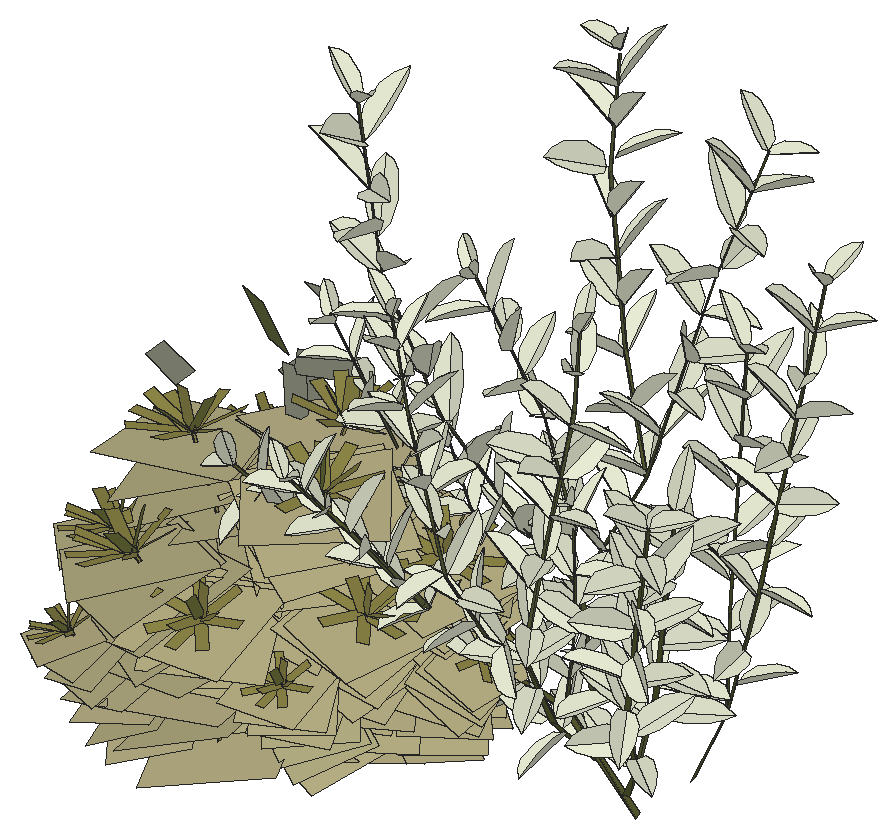
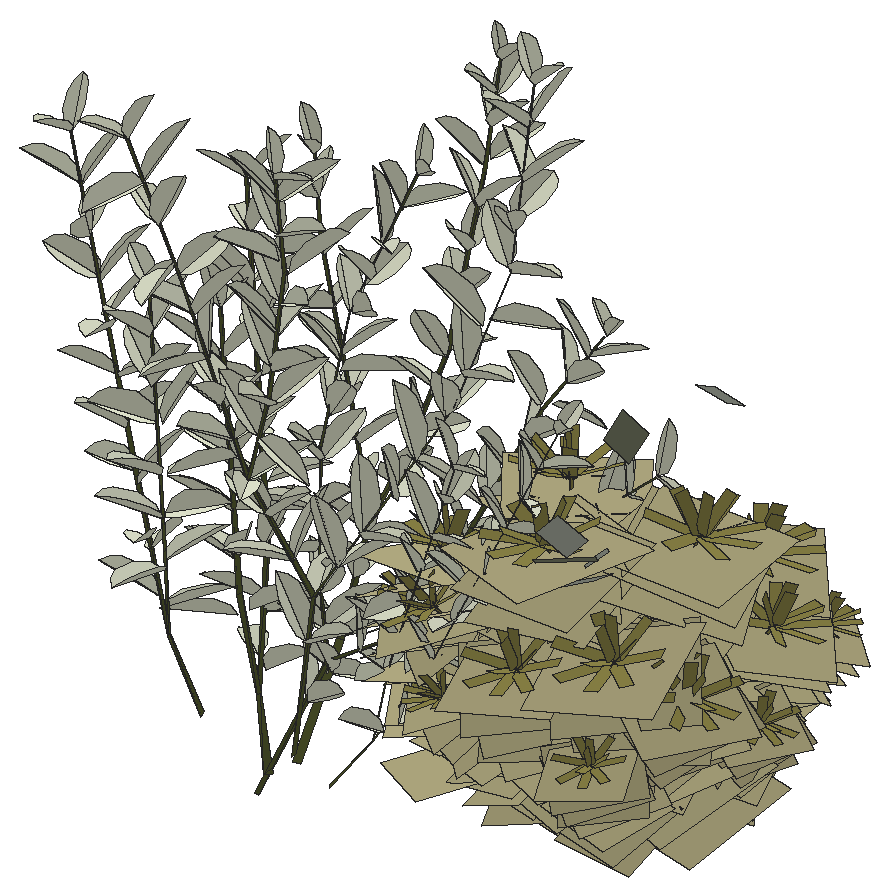
# SketchUp Ruby script. Lengths in inches.
U = 1.inch
M = Sketchup.active_model
def pt(a) = Geom::Point3d.new(a.map { |v| v * U })
def face(e, loops, mat)
  f = e.add_face(loops[0].map { |a| pt(a) })
  loops[1..].each { |l| e.add_face(l.map { |a| pt(a) }).erase! }
  f.material = f.back_material = mat if mat
  f
end
# faces: each face lists its corners as indices into pts; further lists are holes
def faces(e, pts, list, mat = nil) = list.each { |f| face(e, (f[0].is_a?(Array) ? f : [f]).map { |l| l.map { |i| pts[i] } }, mat) }
# xy, xz, yz: faces in a plane at the given z, y or x. An outline is a flat list of corners, or four numbers for a rectangle; further outlines are holes
def ring(l) = l.size == 4 ? [[l[0], l[1]], [l[2], l[1]], [l[2], l[3]], [l[0], l[3]]] : l.each_slice(2).to_a
def flat(e, list, mat, &to3) = list.each { |f| face(e, (f[0].is_a?(Array) ? f : [f]).map { |l| ring(l).map { |u, v| to3.(u, v) } }, mat) }
def xy(e, z, list, mat = nil) = flat(e, list, mat) { |x, y| [x, y, z] }
def xz(e, y, list, mat = nil) = flat(e, list, mat) { |x, z| [x, y, z] }
def yz(e, x, list, mat = nil) = flat(e, list, mat) { |y, z| [x, y, z] }
def lines(e, pts, list) = list.each { |a, b| e.add_line(pt(pts[a]), pt(pts[b])) }
# prism: a flat outline (further loops are holes) pulled along v
def prism(e, loops, v, mat = nil)
  f = face(e, loops, mat); d = Geom::Vector3d.new(v.map { |x| x * U })
  f.pushpull(f.normal.samedirection?(d) ? d.length : -d.length)
end
def box(e, o, s, mat = nil) = prism(e, [[o, [o[0] + s[0], o[1], o[2]], [o[0] + s[0], o[1] + s[1], o[2]], [o[0], o[1] + s[1], o[2]]]], [0, 0, s[2]], mat)
def at(x, y, z, deg = 0) = Geom::Transformation.translation(pt([x, y, z])) * Geom::Transformation.rotation(ORIGIN, Z_AXIS, deg.degrees)
def axes(o, x, y, z) = Geom::Transformation.new([*x, 0, *y, 0, *z, 0, *pt(o).to_a, 1])
def part(name) = M.definitions.add(name)
# library, detail: a bought-in or finely detailed component or shape, given as its bounding box
def library(name, o, s) = part(name).tap { |d| box(d.entities, o, s) }
def detail(e, o, s) = box(e.add_group.entities, o, s)
def put(e, d, t, mat = nil) = e.add_instance(d, t).tap { |i| i.material = mat if mat }
def group(e, t, mat = nil) = e.add_group.tap { |g| g.transformation = t; g.material = mat if mat }.entities
root = M.entities
M.materials.add("0ad16as01f6asdLeafVar1sfd015as60f1as6").color = [231, 235, 211]
M.materials.add("Colorsadfasdfa0sd1f06w3").color = [153, 130, 61]
M.materials.add("Euphorbia asdfasd0f150160s159w").color = [180, 173, 131]
M.materials.add("Euphorbiaasdfa0sdf1a56sd016wow Leaf SU").color = [141, 134, 72]
M.materials.add("asdfasdf0165f6asdLeafVar1sfd015as60f1as6").color = [231, 235, 211]
M.materials.add("dw_stemssadfasdfa0sdf1s01d6w1").color = [90, 97, 50]
M.materials.add("viburnumblaasdfas0df1w06d").color = [98, 102, 84]
M.materials.add("viburnumbladsadfasdfad0w122").color = [125, 129, 119]
c1 = part("Component\#315")
p = [[0.25,0,0],[2.05,0.01,0.35],[1.81,4.2,1.66],[0,4.19,1.3125]]
faces(c1.entities,p,[[0,1,2,3]],"viburnumbladsadfasdfad0w122")
c2 = part("viburnumblad2")
put(c2.entities,c1,axes([-19.23,-4.49,-32.18],[83.35428,0,0],[0,79.38502,0],[0,0,83.35428]))
c3 = part("Component\#314")
p = [[0.14,0,0],[2.58,0.05,0.25],[2.44,5.11,2.64],[0,5.05,2.39]]
faces(c3.entities,p,[[0,1,2,3]],"viburnumblaasdfas0df1w06d")
c4 = part("viburnumblad1\#2")
put(c4.entities,c3,axes([-37.25,6.23,19.31],[75.98784,0,0],[0,65.50676,0],[0,0,75.98784]))
c5 = part("Component\#306")
p = [[4.55,0.11,0],[4.55,0,0],[2.84,0,3.13],[2.84,0.11,3.13],[4.625,0.05,0.04],[2.92,0.05,3.15],
  [2.08,0,8.07],[2.08,0.11,8.07],[2.16,0.05,8.1],[0,0,12.54],[0,0.11,12.54],[0.07,0.05,12.58]]
faces(c5.entities,p,[[0,1,2,3],[1,4,5,2],[1,0,4],[4,0,3,5],[3,2,6,7],[2,5,8,6],[5,3,7,8],[7,6,9,10],
  [6,8,11,9],[8,7,10,11],[10,9,11]],"Colorsadfasdfa0sd1f06w3")
c6 = part("Component\#301")
xy(c6.entities,0,[[0,0,0.7,3.1]],"Euphorbiaasdfa0sdf1a56sd016wow Leaf SU")
c7 = part("Leaf rosette")
put(c7.entities,c6,axes([2.21,1.74,0.13],[-0.4441,0.47879,-0.0956],[-0.4878,-0.4406,0.05935],[-0.03146,0.16757,0.98536]))
put(c7.entities,c6,axes([2.29,1.9,0.17],[-0.62678,-0.10063,-0.18061],[0.01105,-0.59203,0.2915],[-0.31282,0.41486,0.85442]))
put(c7.entities,c6,axes([2.09,1.69,0.1],[-0.10438,0.65169,0],[-0.65169,-0.10438,0],[0,0,1]))
put(c7.entities,c6,axes([1.97,1.77,0.02],[0.31114,0.5228,0.25587],[-0.57125,0.32993,0.02052],[-0.16918,-0.3502,0.92127]))
put(c7.entities,c6,axes([1.93,1.95,0],[0.54816,-0.03215,0.36617],[-0.11878,0.60671,0.23108],[-0.52706,-0.39065,0.75472]))
put(c7.entities,c6,axes([2.04,2.1,0.05],[0.26275,-0.55867,0.23335],[0.34186,0.34684,0.44545],[-0.75711,-0.08556,0.64766]))
put(c7.entities,c6,axes([2.22,2.08,0.13],[-0.29265,-0.59104,-0.02512],[0.40323,-0.2198,0.47401],[-0.65583,0.2952,0.69479]))
c8 = part("Component\#308")
xy(c8.entities,0,[[0,0,5.01,4.64]],"Euphorbia asdfasd0f150160s159w")
c9 = part("Component\#316")
put(c9.entities,c5,at(2.35,3.5,0))
put(c9.entities,c7,at(0.25,1.59,12.45))
put(c9.entities,c8,axes([7.46,0.77,3.64],[0.10848,0.99337,0.03799],[-0.82378,0.11122,-0.55589],[-0.55643,0.02901,0.83038]))
put(c9.entities,c8,axes([1.97,2.58,1.93],[0.80762,-0.50565,0.30344],[0.47433,0.86274,0.17519],[-0.35038,0.00244,0.93661]))
put(c9.entities,c8,axes([5.79,0.14,3.9],[0.5013,0.78918,0.35482],[-0.74775,0.60146,-0.2813],[-0.4354,-0.1243,0.89162]))
put(c9.entities,c8,axes([1.87,2.6,3.75],[0.73154,-0.49698,0.46676],[0.47433,0.86274,0.17519],[-0.48976,0.09324,0.86686]))
put(c9.entities,c8,axes([3.91,7.06,6.66],[-0.50827,-0.83837,-0.19699],[0.8278,-0.53869,0.15675],[-0.23753,-0.08339,0.96779]))
put(c9.entities,c8,axes([1.2,3.99,6.83],[0.56066,-0.79708,0.22433],[0.74237,0.60386,0.29025],[-0.36682,0.0038,0.93028]))
put(c9.entities,c6,axes([2.42,3.73,12.57],[-0.1322,-0.64472,0.04955],[0.10064,0.02944,0.65162],[-0.9678,0.2092,0.14002]))
put(c9.entities,c6,axes([2.57,3.43,12.63],[-0.62833,0.089,-0.18134],[-0.19954,-0.36568,0.51192],[-0.04764,0.82148,0.56824]))
put(c9.entities,c8,axes([4.04,6.92,11.09],[-0.67411,-0.5063,-0.5378],[0.44628,-0.85937,0.24964],[-0.58857,-0.07172,0.80526]))
put(c9.entities,c6,axes([2.5,3.49,12.74],[-0.62833,0.089,-0.18134],[-0.18746,-0.03618,0.63178],[0.11402,0.98935,0.09049]))
put(c9.entities,c6,axes([2.3,3.27,12.51],[0.02916,0.64747,0.12464],[-0.56235,-0.04072,0.34308],[0.5216,-0.18387,0.83314]))
put(c9.entities,c8,axes([0.26,4.96,9.69],[0.33661,-0.92735,0.16343],[0.73504,0.36725,0.56995],[-0.58857,-0.07172,0.80526]))
put(c9.entities,c8,axes([4.76,6.31,12.62],[-0.95056,-0.1129,-0.28929],[0.09021,-0.99179,0.09066],[-0.29715,0.06008,0.95294]))
put(c9.entities,c8,axes([5.2,6.55,10.37],[-0.76372,-0.27738,-0.58291],[0.26517,-0.95808,0.10848],[-0.58857,-0.07172,0.80526]))
c10 = part("Plant stem")
p = [[2.84,0.11,3.13],[2.84,0,3.13],[2.08,0,8.07],[2.08,0.11,8.07],[2.92,0.05,3.15],[2.16,0.05,8.1],
  [0,0,12.54],[0,0.11,12.54],[0.07,0.05,12.58]]
faces(c10.entities,p,[[0,1,2,3],[1,4,5,2],[4,0,3,5],[3,2,6,7],[2,5,8,6],[5,3,7,8],[7,6,8]],"Colorsadfasdfa0sd1f06w3")
c11 = part("Leafy shoot")
put(c11.entities,c10,at(2.35,3.5,0))
put(c11.entities,c7,at(0.25,1.59,12.45))
put(c11.entities,c8,axes([1.87,2.6,3.75],[0.73154,-0.49698,0.46676],[0.47433,0.86274,0.17519],[-0.48976,0.09324,0.86686]))
put(c11.entities,c8,axes([3.91,7.06,6.66],[-0.50827,-0.83837,-0.19699],[0.8278,-0.53869,0.15675],[-0.23753,-0.08339,0.96779]))
put(c11.entities,c8,axes([1.2,3.99,6.83],[0.56066,-0.79708,0.22433],[0.74237,0.60386,0.29025],[-0.36682,0.0038,0.93028]))
put(c11.entities,c6,axes([2.42,3.73,12.57],[-0.1322,-0.64472,0.04955],[0.10064,0.02944,0.65162],[-0.9678,0.2092,0.14002]))
put(c11.entities,c6,axes([2.57,3.43,12.63],[-0.62833,0.089,-0.18134],[-0.19954,-0.36568,0.51192],[-0.04764,0.82148,0.56824]))
put(c11.entities,c8,axes([4.04,6.92,11.09],[-0.67411,-0.5063,-0.5378],[0.44628,-0.85937,0.24964],[-0.58857,-0.07172,0.80526]))
put(c11.entities,c6,axes([2.5,3.49,12.74],[-0.62833,0.089,-0.18134],[-0.18746,-0.03618,0.63178],[0.11402,0.98935,0.09049]))
put(c11.entities,c6,axes([2.3,3.27,12.51],[0.02916,0.64747,0.12464],[-0.56235,-0.04072,0.34308],[0.5216,-0.18387,0.83314]))
put(c11.entities,c8,axes([0.26,4.96,9.69],[0.33661,-0.92735,0.16343],[0.73504,0.36725,0.56995],[-0.58857,-0.07172,0.80526]))
put(c11.entities,c8,axes([4.76,6.31,12.62],[-0.95056,-0.1129,-0.28929],[0.09021,-0.99179,0.09066],[-0.29715,0.06008,0.95294]))
put(c11.entities,c8,axes([5.2,6.55,10.37],[-0.76372,-0.27738,-0.58291],[0.26517,-0.95808,0.10848],[-0.58857,-0.07172,0.80526]))
put(c11.entities,c8,axes([7.03,0.77,3.77],[0.19714,0.84663,0.32426],[-0.94994,0.28899,-0.30484],[-0.2731,-0.45173,0.91532]))
c12 = part("Groundcover plant")
put(c12.entities,c9,axes([0.82,1.83,0.8125],[0.98541,0,-0.17021],[0,1,0],[0.17021,0,0.98541]))
put(c12.entities,c11,axes([4.45,-0.84,-2.24],[0.69527,0.50616,0],[-0.50264,0.69042,-0.10135],[-0.05965,0.08194,0.85401]))
put(c12.entities,c11,axes([1.85,7.37,-3.38],[0.7038,-0.47341,0.14191],[0.46407,0.71797,0.09357],[-0.16999,0,0.84303]))
put(c12.entities,c11,axes([6.9,-3.65,-2.52],[0.79351,0.57769,0],[-0.57366,0.78798,-0.11567],[-0.06808,0.09351,0.97468]))
put(c12.entities,c11,axes([1.36,5.18,-2.66],[0.50674,-0.34086,0.10218],[0.33413,0.51694,0.06737],[-0.12239,0,0.60698]))
put(c12.entities,c11,axes([5.76,-1.49,-2.17],[0.43479,0.43181,0.07251],[-0.43488,0.43544,-0.06951],[-0.06212,-0.06169,0.61918]))
c13 = part("Groundcover clump")
put(c13.entities,c12,axes([25.06,6.72,0.82],[-0.74291,1.22188,0],[-1.22188,-0.74291,0],[0,0,1]))
put(c13.entities,c12,axes([-0.76,2.1875,0.82],[1.43,0,0],[0,1.43,0],[0,0,1]))
put(c13.entities,c12,axes([8.21,24.79,0.82],[-0.6403,-1.27864,0],[1.27864,-0.6403,0],[0,0,1]))
c14 = part("vdw_leaf\#3")
p = [[0,0,0],[-2.77,1.61,2.32],[-4.3125,6.1,4.5],[-3.97,13.49,6.09],[-2.47,18.57,6.3],[-0.2,22.73,5.75],
  [2.54,19.66,6.85],[4.3,15.93,7.09],[5.03,7.6,5.43],[3.32,1.76,2.74]]
faces(c14.entities,p,[[0,1,2,3,4,5],[0,5,6,7,8,9]],"asdfasdf0165f6asdLeafVar1sfd015as60f1as6")
c15 = part("dw_brancj_2\#2")
p = [[9.7,-0.22,29.95],[0.23,-1.96,0.34],[-0.05,1.51,0.11],[9.65,1.51,29.46],[18.64,-8.75,84.43],[18.96,-6.63,84.625],
  [1.53,6.02,63.68],[1.42,8.18,63.25],[-10.58,8.77,161.17],[-10.41,9.98,160.68],[26.34,-9.37,211.72],[26.57,-8.28,211.23]]
faces(c15.entities,p,[[0,1,2],[0,2,3],[4,0,3],[4,3,5],[6,0,3],[6,3,7],[8,6,7],[8,7,9],
  [10,4,5],[10,5,11]],"dw_stemssadfasdfa0sdf1s01d6w1")
c16 = part("vdw_branch2\#3")
put(c16.entities,c14,axes([19.53,-5.9,102.42],[1.12377,-0.50004,0],[0.46097,1.03596,0.47664],[-0.19377,-0.43548,1.13389]))
put(c16.entities,c14,axes([-5.89,6.52,109.44],[-1.07209,0.83679,0],[-0.77141,-0.98832,0.52702],[0.32427,0.41545,1.25373]))
put(c16.entities,c14,axes([-0.44,8.23,75.28],[0.88709,-0.9947,0],[0.92159,0.82189,0.33087],[-0.25219,-0.22491,1.26111]))
put(c16.entities,c14,axes([24.71,-8.97,190.81],[-0.82641,0.91101,0],[-0.83983,-0.76184,0.47664],[0.35303,0.32025,1.13389]))
put(c16.entities,c14,axes([-2.29,8.24,91.35],[1.24603,-0.47303,0],[0.43826,1.15445,0.33087],[-0.11993,-0.31592,1.26111]))
put(c16.entities,c14,axes([12.26,-3.11,37.92],[-0.64625,1.02205,0.22511],[-1.04383,-0.61044,-0.22511],[-0.07533,-0.30931,1.18809]))
put(c16.entities,c14,axes([26.17,-9.17,210.27],[-0.99452,-0.10453,0],[0.09636,-0.91681,0.38752],[-0.04051,0.38539,0.92186]))
put(c16.entities,c14,axes([-6.07,9.4,125.35],[-0.90214,-0.98107,0],[0.90896,-0.83583,0.33087],[-0.24874,0.22873,1.26111]))
put(c16.entities,c14,axes([-4.13,7.29,110.58],[0.44715,-1.078,0.64369],[1.05816,0.63649,0.33087],[-0.58725,0.40856,1.09216]))
put(c16.entities,c14,axes([23.91,-8.22,171.96],[0.62307,0.85009,-0.63406],[-0.71531,0.8798,0.47664],[0.78296,0.12729,0.94004]))
put(c16.entities,c15,at(-0.09,0.18,-0.25),"dw_stemssadfasdfa0sdf1s01d6w1")
put(c16.entities,c14,axes([23.34,-9.65,156.59],[-0.31364,-1.00782,0.58216],[1.10369,-0.17062,0.29925],[-0.17137,0.6239,0.98776]))
put(c16.entities,c14,axes([15.03,-3.37,58.83],[-1.05425,-0.00194,0.58442],[-0.14303,-1.11707,-0.26172],[0.55355,-0.3046,0.99755]))
put(c16.entities,c14,axes([-11.625,9.46,160.37],[0.36812,0.92978,0],[-0.85713,0.33936,0.38752],[0.3603,-0.14265,0.92186]))
put(c16.entities,c14,axes([21.32,-8.53,138.72],[1.21379,0.19904,0],[-0.19904,1.21379,0],[0,0,1.23]))
put(c16.entities,c14,axes([22.54,-9.2,141.43],[-1.02887,0.17955,0.60182],[-0.23387,-1.13057,-0.06253],[0.56696,-0.17376,1.02111]))
put(c16.entities,c14,axes([23.9,-8.82,173.84],[-1.14567,-0.37474,0],[0.35918,-1.0981,0.04438],[-0.01409,0.04308,1.17993]))
put(c16.entities,c14,axes([-7.84,8.92,143.59],[-1.26971,0.40522,0],[-0.37543,-1.17638,0.33087],[0.10274,0.32192,1.26111]))
put(c16.entities,c14,axes([19.77,-8.01,85.98],[-0.32405,-1.14591,0.18674],[1.10278,-0.32969,-0.10948],[0.15845,0.14442,1.16117]))
put(c16.entities,c14,axes([-0.62,5.76,76.34],[-0.08879,1.17576,-0.67771],[-1.34525,-0.16582,-0.11144],[-0.17897,0.66309,1.17383]))
put(c16.entities,c14,axes([20.49,-8.22,121.07],[0.39924,-0.78471,-0.8233],[1.08735,0.33121,0.2116],[0.09035,-0.83005,0.83495]))
put(c16.entities,c14,axes([15.15,-3.72,62.9],[1.16251,0.40128,-0.0211],[-0.39924,1.16074,0.07874],[0.0456,-0.06757,1.2273]))
put(c16.entities,c14,axes([20.72,-8.08,120.26],[-0.03693,1.2277,-0.06551],[-1.22944,-0.03698,0],[-0.00197,0.06548,1.22825]))
put(c16.entities,c14,axes([22.58,-8.36,155.57],[-0.56247,1.09386,0],[-1.00839,-0.51852,0.47664],[0.42389,0.21796,1.13389]))
put(c16.entities,c14,axes([3.97,3.13,57.96],[-1.09459,0.76041,0],[-0.72262,-1.0402,-0.1735],[-0.10109,-0.14552,1.29352]))
put(c16.entities,c14,axes([-10.8,9.06,160.75],[-0.66334,-0.72138,0],[0.66835,-0.61458,0.24329],[-0.1829,0.16818,0.92729]))
put(c16.entities,c14,axes([19.06,-9.3125,103.96],[-1.01345,0.25553,-0.60051],[-0.2265,-1.12952,-0.09839],[-0.59598,0.03076,1.01889]))
put(c16.entities,c14,axes([18.07,-6.2,81.7],[-0.56247,1.09386,0],[-1.00839,-0.51852,0.47664],[0.42389,0.21796,1.13389]))
put(c16.entities,c14,axes([12.95,-0.39,43.31],[0.13044,-1.19832,0],[1.11025,0.12085,0.29925],[-0.30382,-0.03307,1.14057]))
put(c16.entities,c14,axes([2.28,8.28,56.18],[1.32413,-0.31027,0],[0.30923,1.31968,-0.11144],[0.02542,0.1085,1.35543]))
put(c16.entities,c14,axes([-7.55,9.96,143.07],[1.34251,-0.21744,0],[0.20045,1.23761,0.52702],[-0.08426,-0.52024,1.25373]))
put(c16.entities,c14,axes([26.15,-8.25,210.66],[0.94661,-0.25364,0],[0.235,0.87703,0.24329],[-0.06431,-0.24,0.92729]))
put(c16.entities,c14,axes([-6.48,11.37,125.16],[0.64635,1.10315,0.46356],[-1.16569,0.46153,0.52702],[0.27017,-0.6478,1.16488]))
put(c16.entities,c14,axes([25.74,-8.35,191.28],[0.13044,-1.19832,0],[1.11025,0.12085,0.29925],[-0.30382,-0.03307,1.14057]))
put(c16.entities,c14,axes([-5.125,7.47,91.6],[-1.10024,0.63688,0.48318],[-0.78682,-1.00808,-0.46292],[0.14137,-0.65404,1.184]))
c17 = part("vdw_leaf\#1")
p = [[0,0,0],[-2.77,1.61,2.32],[-4.3125,6.1,4.5],[-3.97,13.49,6.09],[-2.47,18.57,6.3],[-0.2,22.73,5.75],
  [2.54,19.66,6.85],[4.3,15.93,7.09],[5.03,7.6,5.43],[3.32,1.76,2.74]]
faces(c17.entities,p,[[0,1,2,3,4,5],[0,5,6,7,8,9]],"0ad16as01f6asdLeafVar1sfd015as60f1as6")
c18 = part("dw_branch_3\#2")
p = [[-10.06,-1.6,62.9],[-0.2,1.54,-0.01],[-10.43,1.54,62.72],[0.18,-1.6,0.17],[-23.75,-21.66,88.91],[-25.7,-20.3,89.55],
  [13.4,11.62,104.56],[13.33,13.52,104.47],[-49.25,-41.87,130.3125],[-50.33,-40.21,130.71],[-4.97,21.13,143.98],[35.61,27.99,178.64],
  [-5.09,23.64,143.96],[35.32,29.14,178.46],[-67.7,-55.38,181.06],[-68.34,-54.45,181.62],[-22.8125,33.9,200.59],[-22.94,35.79,200.41],
  [56.61,36.78,229.75],[56.29,38.09,229.57],[-70.63,-67.46,248.85],[-70.72,-66.33,249.5],[-25.05,43.32,240.75],[-24.98,44.26,240.57]]
faces(c18.entities,p,[[0,1,2],[0,3,1],[4,2,5],[4,0,2],[6,0,2],[6,2,7],[8,4,5],[8,5,9],
  [10,6,7],[11,6,7],[10,7,12],[11,7,13],[14,8,9],[14,9,15],[16,10,12],[16,12,17],
  [18,11,13],[18,13,19],[20,14,15],[20,15,21],[22,16,17],[22,17,23]],"dw_stemssadfasdfa0sdf1s01d6w1")
c19 = part("dw_branch3\#2")
put(c19.entities,c17,axes([-70.33,-63.58,233.32],[-1.00752,0.412,0.78596],[-0.24851,-1.22189,0.32195],[0.83141,0.09817,1.01433]))
put(c19.entities,c17,axes([-66.93,-54.91,182.82],[-0.84976,-0.98359,0.33619],[0.99572,-0.74889,0.32577],[-0.05223,0.46521,1.22907]))
put(c19.entities,c17,axes([-46.12,-39.49,126.35],[1.23843,0.5364,0.23552],[-0.56438,0.94474,0.81599],[0.15707,-0.83465,1.07498]))
put(c19.entities,c17,axes([13.0625,13.13,104.77],[-1.01271,0.69982,-0.26884],[-0.74268,-0.99813,0.19939],[-0.10222,0.31872,1.21473]))
put(c19.entities,c17,axes([-18.87,30.42,186.42],[0.36309,1.06515,-0.56675],[-1.14134,0.49515,0.19939],[0.39128,0.45593,1.10754]))
put(c19.entities,c17,axes([-3.2,4.15,75.77],[-1.04153,0.55414,0.44243],[-0.23365,-1.01045,0.71554],[0.6695,0.50943,0.93801]))
put(c19.entities,c17,axes([23.2,19.41,136.3],[-0.65687,-1.11295,-0.05714],[1.05857,-0.61429,-0.20411],[0.15163,-0.1536,1.24868]))
put(c19.entities,c17,axes([-25.57,35.48,201.32],[-0.64726,0.62827,0.87973],[-0.71635,-1.0172,0.19939],[0.80962,-0.39773,0.87973]))
put(c19.entities,c17,axes([-36.37,-32.14,110.35],[-0.80747,1.09962,0.12544],[-0.83333,-0.50188,-0.96467],[-0.72833,-0.64487,0.96467]))
put(c19.entities,c17,axes([-9.89,26.72,156.79],[0.45529,1.02969,0.56572],[-1.16919,0.33753,0.32662],[0.11537,-0.64297,1.07744]))
put(c19.entities,c17,axes([-26.57,46.1,241.0625],[0.00015,0.80921,0.22536],[-0.83985,0.00446,-0.01542],[-0.01605,-0.22532,0.80906]))
put(c19.entities,c17,axes([-9.2,-2.58,61.06],[-1.10001,-0.40312,0.39014],[0.40883,-1.1116,0.00411],[0.35732,0.13566,1.14763]))
put(c19.entities,c17,axes([-69.91,-63.11,233.93],[1.36249,-0.1432,0],[0.13201,1.25603,0.5309],[-0.05549,-0.52799,1.26295]))
put(c19.entities,c17,axes([32.2,25.46,166.13],[0.06878,-1.29051,-0.05714],[1.22165,0.07415,-0.20411],[0.2113,-0.04403,1.24868]))
put(c19.entities,c17,axes([-5.68,-0.66,44.43],[-0.48448,-1.12287,0.17078],[0.98138,-0.33653,0.57135],[-0.48308,0.36756,1.04626]))
put(c19.entities,c17,axes([43.45,32.81,198.64],[0.5408,1.19584,0.14106],[-0.94242,0.32409,0.86557],[0.74952,-0.45533,0.98656]))
put(c19.entities,c17,axes([12.52,14.14,104.98],[1.02694,0.54888,0.41092],[-0.53566,1.05407,-0.06927],[-0.38969,-0.12321,1.13846]))
put(c19.entities,c17,axes([44.55,32.375,198.73],[-0.65687,-1.11295,-0.05714],[1.05857,-0.61429,-0.20411],[0.15163,-0.1536,1.24868]))
put(c19.entities,c17,axes([-5.67,21.17,141.44],[-1.10726,0.43603,-0.32953],[-0.49537,-1.03435,0.29588],[-0.17521,0.40597,1.12589]))
put(c19.entities,c17,axes([55.69,37.84,229.48],[0.18984,0.96334,0.18958],[-0.71996,0.0053,0.69399],[0.66755,-0.26823,0.69457]))
put(c19.entities,c17,axes([-21.52,36.85,205.2],[0.72606,-0.98817,0.14519],[0.94364,0.7084,0.10251],[-0.16885,0.05176,1.19664]))
put(c19.entities,c17,axes([-68.51,-56.35,196.07],[1.16319,0.72381,0],[-0.66725,1.0723,0.5309],[0.28049,-0.45075,1.26295]))
put(c19.entities,c18,at(0.01,-0.09,-0.02),"dw_stemssadfasdfa0sdf1s01d6w1")
put(c19.entities,c17,axes([-2.49,5.18,75.91],[0.78614,-0.90346,-0.30078],[0.86953,0.79562,-0.11715],[0.28546,-0.14014,1.16705]))
put(c19.entities,c17,axes([-23.125,-16.22,82.25],[0.32175,1.32576,0.12544],[-1.33153,0.31835,0.05068],[0.01989,-0.13382,1.3633]))
put(c19.entities,c17,axes([-23.75,41.99,230.3],[0.85958,-0.87451,0.14519],[0.66531,0.75721,0.62192],[-0.54076,-0.36226,1.01955]))
put(c19.entities,c17,axes([27.07,22.48,149.34],[0.92952,-0.64745,-0.62467],[0.50188,1.074,-0.36637],[0.71693,0.02135,1.04468]))
put(c19.entities,c17,axes([17.66,16.25,119.93],[-0.91649,0.83891,-0.3601],[-0.87434,-0.77966,0.40896],[0.0492,0.54447,1.14321]))
put(c19.entities,c17,axes([-68.37,-54.54,181.63],[0.32047,1.28399,0.35434],[-1.33153,0.31835,0.05068],[-0.03484,-0.35624,1.32241]))
put(c19.entities,c17,axes([-28.98,-27.1,96.48],[-0.8814,-0.35966,-0.98523],[0.75246,-1.11336,-0.26672],[-0.73065,-0.71272,0.91382]))
put(c19.entities,c17,axes([-15.23,28.43,172.72],[-1.21149,0.11898,0.32517],[-0.09739,-1.25259,0.09551],[0.33228,0.0667,1.21356]))
put(c19.entities,c17,axes([-17.5625,31.23,186.85],[-0.49275,-1.12287,0.14519],[0.95014,-0.33653,0.62192],[-0.53717,0.36756,1.01955]))
put(c19.entities,c17,axes([26.7,21.22,149.39],[-1.00104,0.22334,0.83093],[0.36894,-1.0402,0.72406],[0.77731,0.78134,0.72643]))
put(c19.entities,c17,axes([-31.125,-24.87,97.38],[0.75482,-0.86936,0.69068],[-0.00159,0.80023,1.00899],[-1.08766,-0.58016,0.45842]))
put(c19.entities,c17,axes([-71.21,-66.73,248.67],[0.25207,0.96771,0],[-0.8921,0.23237,0.38752],[0.375,-0.09768,0.92186]))
put(c19.entities,c17,axes([-24.11,41.05,229.55],[-1.11612,0.51924,-0.26884],[-0.56394,-1.10897,0.19939],[-0.15444,0.29694,1.21473]))
put(c19.entities,c17,axes([6.75,8.37,91.63],[-0.33418,-1.12287,0.39014],[1.13558,-0.33653,0.00411],[0.10478,0.36756,1.14763]))
put(c19.entities,c17,axes([-26,45.89,241.63],[-0.26986,-0.70824,-0.32129],[0.56818,-0.39091,0.38449],[-0.49365,-0.09775,0.63011]))
put(c19.entities,c17,axes([3.74,17.32,124.35],[0.22441,1.22913,-0.16274],[-1.07812,0.11178,-0.64246],[-0.61228,0.25367,1.07162]))
put(c19.entities,c17,axes([-5.44,22.27,140.88],[1.2203,0.00475,0.31374],[-0.097,1.20386,0.35905],[-0.29841,-0.37189,1.1663]))
put(c19.entities,c17,axes([-13.79,29.35,173.31],[0.83169,-0.90108,0.14519],[0.68877,0.73594,0.62192],[-0.55187,-0.34509,1.01955]))
put(c19.entities,c17,axes([-16.92,-7.26,72.98],[1.30647,0.30378,-0.27886],[0.07026,0.74892,1.14503],[0.40633,-1.10623,0.69861]))
put(c19.entities,c17,axes([4.8,17.55,125.22],[-0.25598,-1.17842,0.26559],[1.01553,-0.08455,0.60363],[-0.56975,0.35087,1.00767]))
put(c19.entities,c17,axes([5.3125,8.35,91.45],[0.00638,1.22913,-0.27714],[-1.16413,0.11178,0.46895],[0.48205,0.25367,1.13617]))
put(c19.entities,c17,axes([38.12,30.57,183.07],[1.12534,0.26182,-0.63833],[-0.46674,1.18829,-0.33545],[0.5081,0.51169,1.10563]))
put(c19.entities,c17,axes([-70.41,-60.38,214.47],[-0.41425,1.30587,0],[-1.20383,-0.38188,0.5309],[0.50605,0.16053,1.26295]))
put(c19.entities,c17,axes([37.03,28.75,180.67],[-1.12533,0.00102,-0.63799],[-0.00113,-1.2408,0],[-0.62497,0.00057,1.10237]))
put(c19.entities,c17,axes([30.71,25.35,165.96],[-0.1364,1.29314,0.22715],[-1.08768,-0.23921,0.70862],[0.73536,-0.11394,1.09026]))
put(c19.entities,c17,axes([-38.05,-30.84,110.67],[-0.31533,-1.27379,-0.2839],[1.018,-0.40311,0.67794],[-0.74394,-0.05723,1.08307]))
put(c19.entities,c17,axes([50.11,34.45,213.36],[-1.05669,0.74401,-0.05714],[-0.616,-0.82138,0.69675],[0.37221,0.60904,1.04705]))
put(c19.entities,c17,axes([-65.32,-58.78,200.07],[-1.14597,-0.19668,-0.6713],[0.21784,-1.26924,0],[-0.64812,-0.11124,1.139]))
put(c19.entities,c17,axes([-53.2,-43.37,143.59],[-0.72817,-1.09167,-0.2839],[0.82127,-0.72411,0.67794],[-0.71934,0.19815,1.08307]))
put(c19.entities,c17,axes([-61.1,-50.25,163.67],[-0.52887,1.19686,-0.30066],[-1.10762,-0.57104,-0.32484],[-0.42634,0.12264,1.23812]))
put(c19.entities,c17,axes([-54.12,-42.96,142.67],[0.32175,1.32576,0.12544],[-1.33153,0.31835,0.05068],[0.01989,-0.13382,1.3633]))
put(c19.entities,c17,axes([22.03,20.08,132.3],[1.17066,0.5058,-0.34078],[-0.35758,1.16671,0.50333],[0.49407,-0.35407,1.17172]))
put(c19.entities,c17,axes([-8.59,26.04,158.21],[-0.49275,-1.12287,0.14519],[0.95014,-0.33653,0.62192],[-0.53717,0.36756,1.01955]))
put(c19.entities,c17,axes([49.92,34.03,213.7],[1.24742,-0.35176,0.25024],[0.42127,1.159,-0.4708],[-0.09426,0.52477,1.20753]))
put(c19.entities,c17,axes([-70.34,-67.02,249.05],[-0.57048,-0.79684,0],[0.73827,-0.52855,0.24329],[-0.20203,0.14464,0.92729]))
put(c19.entities,c17,axes([56.04,36.81,228.63],[0.33451,-0.90845,-0.15237],[0.87636,0.33365,-0.06538],[0.11487,-0.11636,0.94597]))
put(c19.entities,c17,axes([-69.93,-60.58,214.88],[-0.45293,-0.99272,-0.78227],[1.14635,-0.58199,0.07483],[-0.40282,-0.65636,1.06615]))
put(c19.entities,c17,axes([-16.77,-8.59,72.7],[-1.22785,0.11509,0.53076],[-0.24879,-1.22495,-0.30991],[0.46742,-0.38989,1.16587]))
put(c19.entities,c17,axes([18.29,17.18,119.24],[1.19981,-0.45946,0.3029],[0.40159,1.22775,0.27158],[-0.37626,-0.1547,1.25575]))
put(c19.entities,c17,axes([-6.73,-0.68,43.74],[0.05346,1.22913,-0.27201],[-1.22696,0.11178,0.26396],[0.28163,0.25367,1.20164]))
put(c19.entities,c17,axes([-58.57,-48.42,160.98],[0.43385,-1.23789,0.39533],[1.04879,0.57965,0.66404],[-0.76727,0.09236,1.13122]))
put(c19.entities,c17,axes([-23.4,38.49,215.38],[0.06762,1.22913,-0.26884],[-1.23909,0.11178,0.19939],[0.21835,0.25367,1.21473]))
put(c19.entities,c17,axes([-22.21,-16.62,83.17],[-0.72817,-1.09167,-0.2839],[0.82127,-0.72411,0.67794],[-0.71934,0.19815,1.08307]))
put(c19.entities,c17,axes([-45.7,-40.77,126.53],[-1.33715,-0.0713,-0.0976],[0.07167,-1.28508,-0.04314],[-0.09306,-0.0492,1.31098]))
put(c19.entities,c17,axes([-22.39,38.51,216.12],[-0.49275,-1.12287,0.14519],[0.95014,-0.33653,0.62192],[-0.53717,0.36756,1.01955]))
c20 = part("vdw_leaf\#2")
p = [[0,0,0],[-2.77,1.61,2.32],[-4.3125,6.1,4.5],[-3.97,13.49,6.09],[-2.47,18.57,6.3],[-0.2,22.73,5.75],
  [2.54,19.66,6.85],[4.3,15.93,7.09],[5.03,7.6,5.43],[3.32,1.76,2.74]]
faces(c20.entities,p,[[0,1,2,3,4,5],[0,5,6,7,8,9]],"asdfasdf0165f6asdLeafVar1sfd015as60f1as6")
c21 = part("dg_branch_1\#2")
p = [[46.12,1.57,35.62],[46,5.42,35.41],[0.14,1.79,0.05],[0.26,-2.0625,0.27],[74.05,2.99,75.8],[74.11,5.28,75.58],
  [103.46,0.47,94.74],[104.03,2.92,94.84],[81.14,16.92,120.46],[81.2,18.78,120.24],[130.47,-5.6875,130.27],[130.58,-3.66,129.85],
  [80.82,34.4375,191.22],[80.64,35.93,190.9],[148.49,-14.56,203.24],[148.9,-12.8125,203.11],[81.08,37.95,226.93],[81.4,39.1,227.03],
  [157.45,-18.19,250.77],[157.7,-17.01,250.41]]
faces(c21.entities,p,[[0,1,2,3],[4,0,1],[4,1,5],[6,4,5],[6,5,7],[8,4,5],[8,5,9],[10,6,7],
  [10,7,11],[12,8,9],[12,9,13],[14,10,11],[14,11,15],[16,12,13],[16,13,17],[18,14,15],
  [18,15,19]],"dw_stemssadfasdfa0sdf1s01d6w1")
c22 = part("vdw_branch1\#3")
put(c22.entities,c20,axes([120.69,-2.42,117.31],[1.12221,-0.24063,-0.65809],[0.19207,1.24776,-0.12871],[0.65778,0.01392,1.11658]))
put(c22.entities,c20,axes([81,38.9,226.05],[0.7888,-0.58155,0],[0.48308,0.65523,0.47],[-0.28484,-0.38635,0.83138]))
put(c22.entities,c20,axes([78.08,12.69,106.05],[-1.43826,-0.02353,-0.03177],[0.0088,-1.31777,0.57755],[-0.03854,0.57714,1.31741]))
put(c22.entities,c20,axes([130.18,-4.73,130.41],[-0.38031,-1.29044,-0.11242],[1.20662,-0.31032,-0.51987],[0.47109,-0.24694,1.24081]))
put(c22.entities,c20,axes([157.08,-17.89,249.93],[-0.91355,0.40674,0],[-0.37496,-0.84216,0.38752],[0.15762,0.35401,0.92186]))
put(c22.entities,c20,axes([90.64,3.03,86.49],[0.32514,-0.85045,-0.99675],[0.69523,0.98247,-0.61148],[1.11061,-0.36604,0.67459]))
put(c22.entities,c20,axes([80.15,28.42,160.95],[-0.16039,0.95636,-1.06292],[-1.41646,0.03966,0.24943],[0.19509,1.07422,0.93709]))
put(c22.entities,c20,axes([126.74,-5.45,129.22],[-0.59819,0.96152,-0.6841],[-0.85772,0.12575,0.92675],[0.75427,0.88089,0.57856]))
put(c22.entities,c20,axes([133.22,-6.12,150.66],[-0.93823,0.76985,0.59124],[-0.47726,-1.08188,0.65135],[0.84525,0.24366,1.02405]))
put(c22.entities,c20,axes([80.43,22.89,141.32],[-1.42571,-0.19312,0.01373],[0.18338,-1.31425,0.5561],[-0.0621,0.5528,1.32692]))
put(c22.entities,c20,axes([33.14,0.88,26.42],[-0.13338,1.31536,0.04876],[-1.04528,-0.13221,0.7073],[0.72315,0.03348,1.07497]))
put(c22.entities,c20,axes([152.63,-15.08,221.76],[-1.28188,0.41945,0.0579],[-0.3638,-1.18547,0.53367],[0.21665,0.49113,1.23869]))
put(c22.entities,c20,axes([80.05,28.28,160.33],[-0.46732,-1.26661,0.40679],[1.27397,-0.40257,0.21004],[-0.07408,0.44645,1.30501]))
put(c22.entities,c20,axes([153.95,-14.8,235.875],[0.39005,1.07743,0.20605],[-0.96443,0.25296,0.50293],[0.42961,-0.3464,0.99807]))
put(c22.entities,c20,axes([80.2,24.22,141.74],[1.33062,-0.46576,0.02628],[0.44746,1.2746,-0.06608],[-0.00197,0.0722,1.37936]))
put(c22.entities,c20,axes([145.48,-12.5,188.92],[-1.32952,0.16983,0.16138],[-0.09299,-1.2361,0.53471],[0.21503,0.51548,1.22904]))
put(c22.entities,c20,axes([139.64,-9.18,171.24],[0.05682,1.30088,0.23414],[-1.13176,-0.05343,0.57151],[0.58357,-0.22963,1.13417]))
put(c22.entities,c20,axes([70.95,4.35,71.98],[-1.1081,-0.41873,0.64752],[0.33675,-1.28259,-0.25313],[0.6937,-0.04625,1.15721]))
put(c22.entities,c20,axes([59.85,4.55,56.17],[-0.26797,1.24526,0.35754],[-0.9369,-0.41634,0.74783],[0.83377,-0.10389,0.98674]))
put(c22.entities,c20,axes([33.11,3.36,25.66],[-0.57817,-1.07968,-0.5679],[1.11554,-0.21356,-0.7297],[0.49375,-0.78178,0.98363]))
put(c22.entities,c21,at(-0.21,0.34,-0.17),"dw_stemssadfasdfa0sdf1s01d6w1")
put(c22.entities,c20,axes([80.91,19.01,122.53],[-0.84258,1.13222,-0.27981],[-1.15093,-0.75138,0.42537],[0.18861,0.47293,1.3457]))
put(c22.entities,c20,axes([119.8,-1.22,114.1],[-1.3235,-0.25012,0.09101],[0.25933,-1.31572,0.15537],[0.05991,0.1698,1.33794]))
put(c22.entities,c20,axes([46.29,5.1,38.04],[0.98937,0.73827,-0.47585],[-0.72359,1.03721,0.10473],[0.44068,0.18581,1.20453]))
put(c22.entities,c20,axes([81.1875,33.03,184.45],[1.33883,0.26986,0.35053],[-0.09581,1.22087,-0.57399],[-0.42216,0.53228,1.20262]))
put(c22.entities,c20,axes([80.16,36.28,206.98],[-0.83993,0.85737,-0.6234],[-1.05964,-0.65701,0.5241],[0.02941,0.81391,1.07976]))
put(c22.entities,c20,axes([154.86,-16.15,234.87],[0.02509,-1.15302,-0.28506],[1.1487,-0.04894,0.29908],[-0.30202,-0.28195,1.11384]))
put(c22.entities,c20,axes([108.77,-0.33,101.14],[-0.47691,-1.03266,-0.72709],[1.25395,-0.29455,-0.40416],[0.15052,-0.81814,1.06325]))
put(c22.entities,c20,axes([89.79,3.01,85.87],[-0.61344,0.75518,0.8965],[-0.17758,-1.01824,0.73622],[1.13385,0.22574,0.58569]))
put(c22.entities,c20,axes([81.56,20.31,123.29],[0.37259,-1.3435,0.21057],[1.29385,0.32364,-0.22445],[0.16906,0.25791,1.34638]))
put(c22.entities,c20,axes([46.45,1.82,36.74],[-0.77883,0.29892,1.0614],[0.19124,-1.24314,0.49044],[1.08598,0.43329,0.67484]))
put(c22.entities,c20,axes([71.37,4.02,72.32],[0.72905,0.81546,-0.74421],[-0.66805,0.98958,0.42988],[0.8391,0.14186,0.97745]))
put(c22.entities,c20,axes([136.59,-5.88,150.53],[0.85845,-0.99897,-0.12437],[0.96526,0.81273,0.13453],[-0.02572,-0.18182,1.28292]))
put(c22.entities,c20,axes([80.375,38.8,225.86],[-0.25178,0.96778,0],[-0.89216,-0.23211,0.38752],[0.37503,0.09757,0.92186]))
put(c22.entities,c20,axes([74.43,7.99,85.38],[-1.05703,0.91669,-0.33543],[-0.95806,-0.87958,0.61531],[0.18697,0.6754,1.25659]))
put(c22.entities,c20,axes([76.57,9.74,89.32],[0.63146,-1.21538,0.33508],[1.18148,0.49387,-0.43517],[0.26321,0.48577,1.26593]))
put(c22.entities,c20,axes([81.6875,36.97,207.4],[0.09422,-1.04424,0.38486],[1.01646,0.1939,0.27727],[-0.33299,0.33382,0.98727]))
put(c22.entities,c20,axes([157.29,-17.17,249.98],[0.50586,-0.50586,0],[0.38853,0.38853,0.41105],[-0.29684,-0.29684,0.56115]))
put(c22.entities,c20,axes([79.92,15.8,106.09],[1.03917,-0.29343,-0.90675],[-0.14587,1.22131,-0.5624],[0.92163,0.5191,0.88824]))
put(c22.entities,c20,axes([61.95,3.88,56.26],[0.41243,-1.28546,0],[1.17466,0.37688,-0.54831],[0.5221,0.16751,1.23363]))
put(c22.entities,c20,axes([151.99,-14.79,208.15],[-0.48571,-1.21723,-0.32393],[1.25386,-0.50033,0],[-0.12005,-0.30087,1.31056]))
put(c22.entities,c20,axes([108.44,0.62,102.22],[0.82183,0.96078,0.38967],[-0.62327,0.08618,1.10203],[0.79141,-0.88661,0.51693]))
put(c22.entities,c20,axes([145.6,-10.56,188.62],[1.03241,-0.02554,-0.82693],[0.3944,1.11584,0.45794],[0.70325,-0.61672,0.89706]))
put(c22.entities,c20,axes([78.59,32.3,183.89],[-1.12675,-0.42036,0.43987],[0.5899,-0.98149,0.57312],[0.14901,0.70693,1.05726]))
put(c22.entities,c20,axes([152.08,-13.42,223.37],[0.79993,-0.44251,-0.69938],[0.68456,0.82615,0.26026],[0.41048,-0.60953,0.85515]))
put(c22.entities,c20,axes([140.71,-8.74,170.55],[0.41903,-1.24177,-0.32393],[1.26224,0.33728,0.33986],[-0.23168,-0.40836,1.26573]))
put(c22.entities,c20,axes([149.25,-12.53,205.78],[1.24456,0.38285,0.23414],[-0.42999,1.04826,0.57151],[-0.02056,-0.62679,1.13417]))
put(root,c2,axes([1244.125,211.57,26.27],[-0.00489,-0.00995,0.00397],[0.00954,-0.00607,-0.00338],[0.00477,0.0019,0.00949]))
put(root,c2,axes([1244.52,193.84,30.06],[-0.00372,-0.00756,-0.00527],[0.01001,-0.00205,-0.00401],[0.00166,-0.0069,0.00731]))
put(root,c2,axes([1244.8,207.86,22.7],[-0.00278,-0.01118,-0.00257],[0.00839,-0.00011,-0.00838],[0.00753,-0.00365,0.00688]))
put(root,c2,axes([1246.22,206.86,22.73],[-0.00715,-0.00814,0.0046],[0.00423,-0.00805,-0.00746],[0.00803,-0.00268,0.00677]))
put(root,c2,axes([1245.37,207.0625,23.91],[0.00322,-0.00766,-0.00823],[0.00813,0.00764,-0.00386],[0.00755,-0.0046,0.00633]))
put(root,c4,axes([1244.95,203.0625,29.11],[-0.00364,-0.00823,0.00913],[0.00776,-0.0108,-0.00665],[0.01031,0.00314,0.00694]))
put(root,c13,axes([1233.86,182.83,1.17],[1.49047,0,0],[0,1.49047,0],[0,0,1.49047]))
put(root,c16,axes([1264.84,210.35,0.89],[-0.10096,-0.0593,-0.07152],[0.0662,-0.11272,0],[-0.05012,-0.02944,0.14408]))
put(root,c19,axes([1271.95,209.17,-2.75],[-0.12304,0.0546,-0.04713],[-0.02701,-0.11428,-0.0937],[-0.06098,-0.05955,0.13659]))
put(root,c19,axes([1269.34,208.55,0.8],[0.1634,0,0],[0,0.1634,0],[0,0,0.20106]))
put(root,c22,axes([1268.89,208.77,0.51],[0.01907,-0.13922,0],[0.13922,0.01907,0],[0,0,0.17291]))
put(root,c16,axes([1271.375,208.7,-1.28],[0.09858,-0.0952,-0.10951],[0.11351,0.11754,0],[0.06402,-0.06182,0.16863]))
put(root,c16,axes([1276.6,209.13,1.63],[0.15791,0.02906,-0.03733],[-0.02958,0.1607,0],[0.02984,0.00549,0.19757]))
